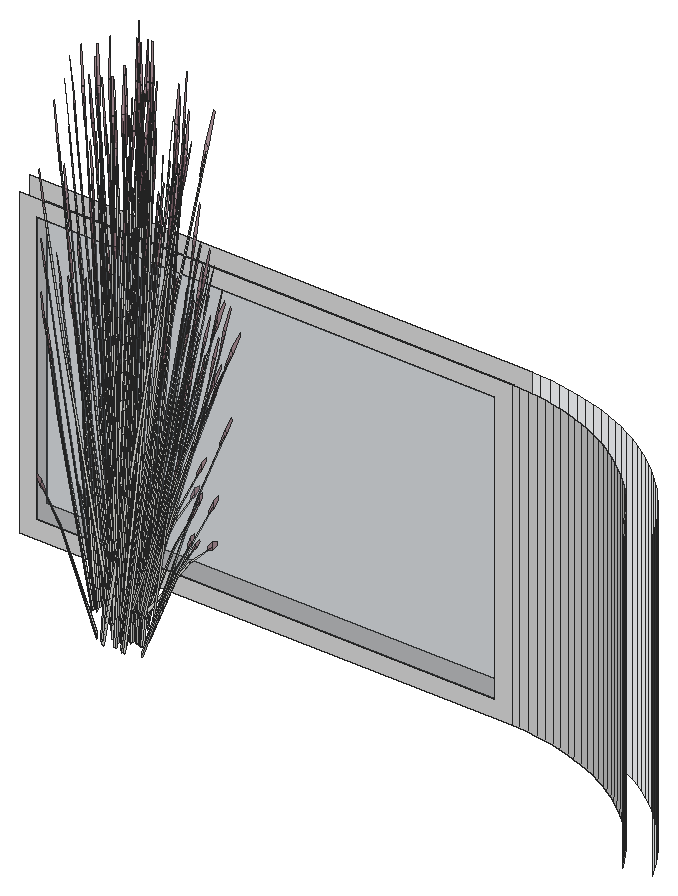
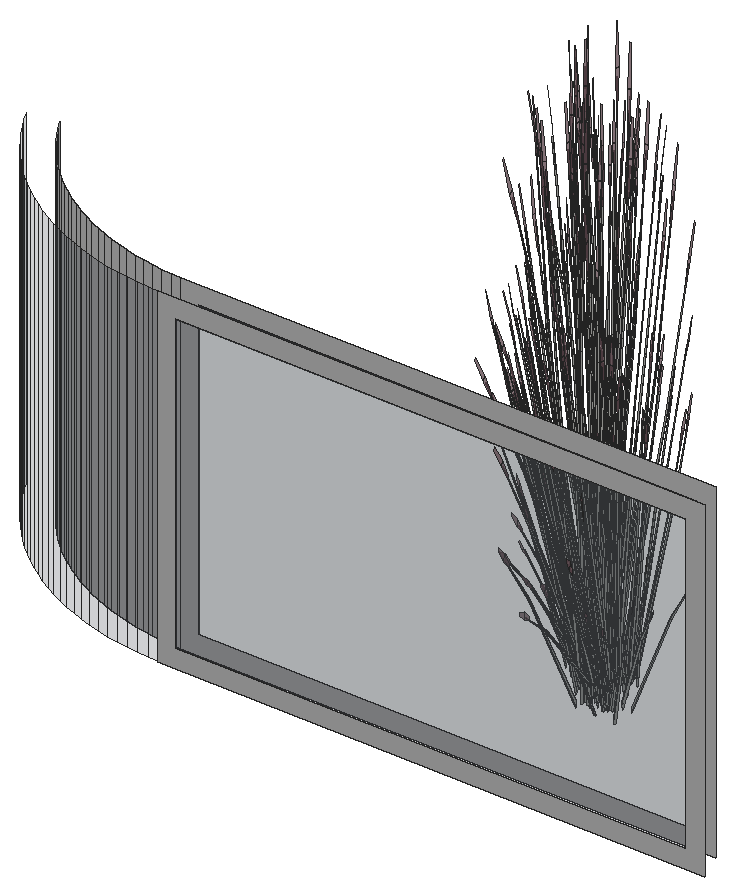
# SketchUp Ruby script. Lengths in inches.
U = 1.inch
M = Sketchup.active_model
def pt(a) = Geom::Point3d.new(a.map { |v| v * U })
def face(e, loops, mat)
  f = e.add_face(loops[0].map { |a| pt(a) })
  loops[1..].each { |l| e.add_face(l.map { |a| pt(a) }).erase! }
  f.material = f.back_material = mat if mat
  f
end
# faces: each face lists its corners as indices into pts; further lists are holes
def faces(e, pts, list, mat = nil) = list.each { |f| face(e, (f[0].is_a?(Array) ? f : [f]).map { |l| l.map { |i| pts[i] } }, mat) }
# xy, xz, yz: faces in a plane at the given z, y or x. An outline is a flat list of corners, or four numbers for a rectangle; further outlines are holes
def ring(l) = l.size == 4 ? [[l[0], l[1]], [l[2], l[1]], [l[2], l[3]], [l[0], l[3]]] : l.each_slice(2).to_a
def flat(e, list, mat, &to3) = list.each { |f| face(e, (f[0].is_a?(Array) ? f : [f]).map { |l| ring(l).map { |u, v| to3.(u, v) } }, mat) }
def xy(e, z, list, mat = nil) = flat(e, list, mat) { |x, y| [x, y, z] }
def xz(e, y, list, mat = nil) = flat(e, list, mat) { |x, z| [x, y, z] }
def yz(e, x, list, mat = nil) = flat(e, list, mat) { |y, z| [x, y, z] }
def lines(e, pts, list) = list.each { |a, b| e.add_line(pt(pts[a]), pt(pts[b])) }
# prism: a flat outline (further loops are holes) pulled along v
def prism(e, loops, v, mat = nil)
  f = face(e, loops, mat); d = Geom::Vector3d.new(v.map { |x| x * U })
  f.pushpull(f.normal.samedirection?(d) ? d.length : -d.length)
end
def box(e, o, s, mat = nil) = prism(e, [[o, [o[0] + s[0], o[1], o[2]], [o[0] + s[0], o[1] + s[1], o[2]], [o[0], o[1] + s[1], o[2]]]], [0, 0, s[2]], mat)
def at(x, y, z, deg = 0) = Geom::Transformation.translation(pt([x, y, z])) * Geom::Transformation.rotation(ORIGIN, Z_AXIS, deg.degrees)
def axes(o, x, y, z) = Geom::Transformation.new([*x, 0, *y, 0, *z, 0, *pt(o).to_a, 1])
def part(name) = M.definitions.add(name)
# library, detail: a bought-in or finely detailed component or shape, given as its bounding box
def library(name, o, s) = part(name).tap { |d| box(d.entities, o, s) }
def detail(e, o, s) = box(e.add_group.entities, o, s)
def put(e, d, t, mat = nil) = e.add_instance(d, t).tap { |i| i.material = mat if mat }
def group(e, t, mat = nil) = e.add_group.tap { |g| g.transformation = t; g.material = mat if mat }.entities
root = M.entities
M.materials.add("Glass_Basic_01").color = [105, 113, 122]
M.materials["Glass_Basic_01"].alpha = 0.25
M.materials.add("LightPink_Translucent").color = [144, 107, 117]
M.materials["LightPink_Translucent"].alpha = 0.75
M.materials.add("M01_Silver_Fog").color = [224, 224, 224]
c1 = part("blade")
p = [[2.15,0.21,22],[0,0.17,0],[0.09,0.45,0],[2.18,0.31,22],[2.29,0.31,22],[0.38,0.45,0],
  [2.48,0.24,33],[2.49,0.24,33],[2.48,0.22,33]]
faces(c1.entities,p,[[0,1,2,3],[4,5,2,3],[6,3,4,7],[8,0,3,6]])
c2 = part("seeds")
p = [[0.3,-0.1,1.38],[-0.01,-0.03,1.59],[-0.01,-0.03,0.03],[0.14,-0.07,-0.07],[0.29,-0.03,3],[0.15,0.01,3.11]]
faces(c2.entities,p,[[0,1,2,3],[1,0,4,5]],"LightPink_Translucent")
c3 = part("blade with seeds")
put(c3.entities,c1,at(0,0,0))
put(c3.entities,c2,axes([2.4,0.25,30.99],[1.5799,-0.05474,1.17369],[-0.12525,1.92788,0.29478],[-0.07173,-0.02425,1.56792]))
xz(root,465.98,[[355.17,648,355.18,684]],"Glass_Basic_01")
xz(root,474,[[275.49,650,329.45,682]],"Glass_Basic_01")
xz(root,474,[[[273.49,648,331.45,684],[275.49,650,329.45,682]]],"M01_Silver_Fog")
xz(root,477,[[274.25,650,329.5,682]],"Glass_Basic_01")
xz(root,477,[[[272.25,648,331.5,684],[274.25,650,329.5,682]]],"M01_Silver_Fog")
yz(root,358.13,[[462.03,648,462.04,684]],"Glass_Basic_01")
p = [[355.6,460.43,648],[356.18,459.47,648],[356.18,459.47,684],[355.6,460.43,684],[359.37,459.91,648],[358.77,460.99,648],
  [358.77,460.99,684],[359.37,459.91,684],[354.98,461.36,648],[354.98,461.36,684],[358.13,462.03,648],[358.13,462.03,684],
  [354.33,462.26,648],[354.33,462.26,684],[358.13,462.04,648],[357.45,463.0625,648],[357.45,463.0625,684],[358.13,462.04,684],
  [353.64,463.14,648],[353.64,463.14,684],[352.92,464,648],[352.92,464,684],[356.73,464.0625,648],[356.73,464.0625,684],
  [352.17,464.83,648],[352.17,464.83,684],[355.97,465.03,648],[355.97,465.03,684],[351.39,465.62,648],[351.39,465.62,684],
  [355.18,465.98,648],[355.18,465.98,684],[350.58,466.39,648],[350.58,466.39,684],[355.17,465.98,648],[354.35,466.89,648],
  [354.35,466.89,684],[355.17,465.98,684],[349.74,467.125,648],[349.74,467.125,684],[353.49,467.76,648],[353.49,467.76,684],
  [348.87,467.83,648],[348.87,467.83,684],[347.97,468.5,648],[347.97,468.5,684],[352.59,468.61,648],[352.59,468.61,684],
  [347.05,469.13,648],[347.05,469.13,684],[351.67,469.42,648],[351.67,469.42,684],[346.11,469.73,648],[346.11,469.73,684],
  [350.71,470.19,648],[350.71,470.19,684],[345.15,470.29,648],[345.15,470.29,684],[349.72,470.93,648],[349.72,470.93,684],
  [344.16,470.82,648],[344.16,470.82,684],[343.16,471.3,648],[343.16,471.3,684],[348.71,471.63,648],[348.71,471.63,684],
  [342.13,471.75,648],[342.13,471.75,684],[347.67,472.29,648],[347.67,472.29,684],[341.09,472.16,648],[341.09,472.16,684],
  [340.04,472.53,648],[340.04,472.53,684],[346.61,472.91,648],[346.61,472.91,684],[338.97,472.86,648],[338.97,472.86,684],
  [337.89,473.15,648],[337.89,473.15,684],[345.52,473.49,648],[345.52,473.49,684],[336.8,473.4,648],[336.8,473.4,684],
  [335.71,473.6,648],[335.71,473.6,684],[344.41,474.03,648],[344.41,474.03,684],[334.6,473.77,648],[334.6,473.77,684],
  [333.49,473.89,648],[333.49,473.89,684],[332.38,473.97,648],[332.38,473.97,684],[331.45,474,648],[331.45,474,684],
  [343.29,474.52,648],[343.29,474.52,684],[342.14,474.97,648],[342.14,474.97,684],[340.98,475.38,648],[340.98,475.38,684],
  [339.8,475.75,648],[339.8,475.75,684],[338.61,476.0625,648],[338.61,476.0625,684],[337.41,476.34,648],[337.41,476.34,684],
  [336.2,476.5625,648],[336.2,476.5625,684],[334.99,476.74,648],[334.99,476.74,684],[333.76,476.88,648],[333.76,476.88,684],
  [332.53,476.97,648],[332.53,476.97,684],[331.5,477,648],[331.5,477,684]]
faces(root,p,[[0,1,2,3],[8,0,3,9],[12,8,9,13],[18,12,13,19],[20,18,19,21],[24,20,21,25],[28,24,25,29],[32,28,29,33],
  [38,32,33,39],[42,38,39,43],[44,42,43,45],[48,44,45,49],[52,48,49,53],[56,52,53,57],[60,56,57,61],[62,60,61,63],
  [66,62,63,67],[70,66,67,71],[72,70,71,73],[76,72,73,77],[78,76,77,79],[82,78,79,83],[84,82,83,85],[88,84,85,89],
  [90,88,89,91],[92,90,91,93],[94,92,93,95]],"M01_Silver_Fog")
faces(root,p,[[4,5,6,7],[5,10,11,6],[14,15,16,17],[15,22,23,16],[22,26,27,23],[26,30,31,27],[34,35,36,37],[35,40,41,36],
  [40,46,47,41],[46,50,51,47],[50,54,55,51],[54,58,59,55],[58,64,65,59],[64,68,69,65],[68,74,75,69],[74,80,81,75],
  [80,86,87,81],[86,96,97,87],[96,98,99,97],[98,100,101,99],[100,102,103,101],[102,104,105,103],[104,106,107,105],[106,108,109,107],
  [108,110,111,109],[110,112,113,111],[112,114,115,113],[114,116,117,115]],"Glass_Basic_01")
put(root,c3,axes([293.05,460.52,652.53],[-0.41757,-0.15024,-0.35414],[0.12179,-0.4383,0.4572],[-0.16812,0.04019,0.87481]))
put(root,c3,axes([291.88,461.33,652.71],[0.06412,0.01444,1.77383],[0.19837,0.47583,-0.16761],[-0.13126,0.12489,0.31391]))
put(root,c3,axes([293.34,460.74,652.68],[-0.13612,0.48987,-0.51099],[-0.46669,-0.16791,-0.3958],[-0.1879,0.04492,0.97773]))
put(root,c3,axes([293.11,460.71,649.49],[0.01274,0.08487,1.76342],[-0.25688,0.44323,-0.26939],[-0.18246,-0.02234,0.30037]))
put(root,c3,axes([292.42,462.84,650.77],[0.2094,-0.24408,1.1486],[0.08263,0.38639,0.84392],[-0.15132,0.06919,0.25299]))
put(root,c3,axes([293.15,460.46,652.73],[0.14195,-0.49104,0.48003],[0.46669,0.16791,0.3958],[-0.18353,0.02951,0.9933]))
put(root,c3,axes([293.32,460.32,653.03],[0.25281,0.48765,-0.1216],[-0.44869,0.23964,-0.67495],[-0.18908,0.06434,1.02557]))
put(root,c3,axes([293.11,460.33,652.73],[-0.18454,-0.3672,0.0643],[0.33652,-0.17973,0.50621],[-0.14834,0.03546,0.77189]))
put(root,c3,axes([293.96,461.35,651.875],[0.1255,-0.16547,1.71376],[0.31687,0.44665,0.13857],[-0.21734,0.2034,0.73262]))
put(root,c3,axes([293.21,461.78,652.53],[-0.43736,0.07697,-0.35414],[-0.11549,-0.43998,0.4572],[-0.12533,0.11818,0.87481]))
put(root,c3,axes([292.97,463.09,649.49],[0.0674,0.0538,1.76342],[0.11428,0.49852,-0.26939],[-0.14937,0.10631,0.30037]))
put(root,c3,axes([293.26,461.6875,652.73],[-0.12461,-0.49565,0.48003],[0.48882,-0.08602,0.3958],[-0.14406,0.11657,0.9933]))
put(root,c3,axes([293.17,461.59,652.73],[-0.34493,-0.22649,0.0643],[0.20082,-0.32253,0.50621],[-0.11059,0.10427,0.77189]))
put(root,c3,axes([293.87,461.76,651.875],[0.09355,-0.18511,1.71376],[0.39247,0.38307,0.13857],[-0.17705,0.23875,0.73262]))
put(root,c3,axes([293.49,460.47,653.05],[0.41757,0.15024,0.35414],[-0.12179,0.4383,-0.4572],[-0.16812,0.04019,0.87481]))
put(root,c3,axes([293.57,461.83,652.68],[0.12908,0.49174,-0.51099],[-0.48882,0.08602,-0.3958],[-0.14008,0.13208,0.97773]))
put(root,c3,axes([292.8,462.72,652.72],[-0.01249,0.10657,1.74944],[0.35444,0.37075,-0.27667],[-0.09279,0.17532,0.14031]))
put(root,c3,axes([294.79,461.48,650.06],[-0.52267,-0.08829,-0.62353],[0.11029,-0.54463,-0.16365],[-0.15598,-0.06599,1.37633]))
put(root,c3,axes([294.1,462.51,650.02],[-0.47024,-0.26927,-0.49651],[0.28107,-0.48284,0],[-0.1071,-0.06133,1.57504]))
put(root,c3,axes([293.34,461.48,653.03],[0.46478,0.29695,-0.1216],[-0.26776,0.43004,-0.67495],[-0.13131,0.14949,1.02557]))
put(root,c3,axes([294.39,462.84,650.375],[-0.31414,0.53965,0],[-0.52557,-0.30095,-0.51607],[-0.1197,-0.06854,1.63711]))
put(root,c3,axes([292.57,462.77,653.65],[0.44338,0.14375,-0.06488],[-0.13639,0.44245,-0.29416],[-0.07252,0.06718,0.97024]))
put(root,c3,axes([293.5625,461.52,653.05],[0.43736,-0.07697,0.35414],[0.11549,0.43998,-0.4572],[-0.12533,0.11818,0.87481]))
put(root,c3,axes([293.8125,463.62,650.59],[0.15856,-0.08496,1.43002],[0.39147,0.25616,-0.30754],[-0.11652,0.22165,0.61141]))
put(root,c3,axes([295.38,461.5625,650.67],[-0.5073,0.35754,-0.29095],[-0.33735,-0.5052,-0.50002],[-0.12516,-0.05131,1.59708]))
put(root,c3,axes([293.98,462.69,652.73],[-0.35779,-0.36745,0.48003],[0.37996,-0.3169,0.3958],[-0.066,0.17239,0.9933]))
put(root,c3,axes([294.23,462.3125,650.03],[-0.11803,-0.46926,-0.30978],[0.46876,-0.13325,0.30978],[-0.0945,-0.05411,1.38974]))
put(root,c3,axes([293.85,462.66,652.73],[-0.4129,-0.02509,0.0643],[0.01132,-0.37891,0.50621],[-0.04321,0.14514,0.77189]))
put(root,c3,axes([293.98,462.8,652.53],[-0.33997,0.28354,-0.35414],[-0.32182,-0.32376,0.4572],[-0.04897,0.1645,0.87481]))
put(root,c3,axes([295.72,461.95,650.06],[-0.33843,0.40479,-0.62353],[-0.42041,-0.36705,-0.16365],[-0.13561,0.10098,1.37633]))
put(root,c3,axes([292.76,463.8125,652.71],[0.057,-0.03251,1.77383],[0.47114,0.21627,-0.16761],[-0.01107,0.18007,0.31391]))
put(root,c3,axes([295.95,461.73,650.46],[-0.49063,-0.43346,-0.25192],[0.41285,-0.48673,0.5513],[-0.13212,0.05071,1.68216]))
put(root,c3,axes([294.2,462.5,653.34],[-0.01307,0.49815,-0.7886],[-0.55054,-0.03346,0.09517],[-0.0581,0.21104,1.11556]))
put(root,c3,axes([294.19,463.9,650.77],[-0.013,-0.32022,1.1486],[0.32493,0.22839,0.84392],[-0.0639,0.15263,0.25299]))
put(root,c3,axes([295.7,461.63,650.21],[-0.54562,0.03324,-0.44739],[-0.04934,-0.55185,0.21531],[-0.09768,0.05593,1.43643]))
put(root,c3,axes([294.66,462.56,650.48],[0.47024,0.26927,0.49651],[-0.28107,0.48284,0],[-0.1071,-0.06133,1.57504]))
put(root,c3,axes([294.02,463.2,651.36],[0.01104,-0.27801,1.54345],[0.49652,0.14685,0.21329],[-0.04302,0.2963,0.72882]))
put(root,c3,axes([295.33,461.72,650.62],[-0.09693,0.48062,0.1448],[-0.47357,-0.08343,-0.41347],[-0.08619,-0.04935,1.26744]))
put(root,c3,axes([296.27,463.06,650.02],[-0.47024,0.26927,-0.49651],[-0.28107,-0.48284,0],[-0.1071,0.06133,1.57504]))
put(root,c3,axes([296.3,462.91,650.19],[-0.31023,-0.54153,-0.05142],[0.52557,-0.30095,0.51607],[-0.12951,0.05156,1.6363]))
put(root,c3,axes([294.3125,462.67,653],[0.35968,0.36185,-0.5672],[-0.37996,0.3169,-0.43934],[-0.05473,0.18385,1.08528]))
put(root,c3,axes([296.16,462.84,650.03],[-0.46876,-0.13325,-0.30978],[0.11803,-0.46926,0.30978],[-0.0945,0.05411,1.38974]))
put(root,c3,axes([294.15,462.4,653.05],[0.33997,-0.28354,0.35414],[0.32182,0.32376,-0.4572],[-0.04897,0.1645,0.87481]))
put(root,c3,axes([296.43,460.84,650.84],[-0.01373,-0.50706,1.41272],[0.62119,0.13144,0.59816],[-0.14692,0.27746,1.3335]))
put(root,c3,axes([293.9375,462.48,653.4],[0.55221,0.02668,-0.13498],[-0.01509,0.50521,-0.74919],[-0.03836,0.19458,1.13838]))
put(root,c3,axes([293.92,463.21,650.82],[0.45645,-0.09537,0.06507],[0.10494,0.38421,-0.86304],[-0.02894,0.19449,0.7736]))
put(root,c3,axes([296.08,461.48,650.67],[0.05855,0.61451,-0.29095],[-0.60981,0.03716,-0.50002],[-0.10738,0.08185,1.59708]))
put(root,c3,axes([294.72,462.15,651.875],[-0.0123,-0.2067,1.71376],[0.53301,0.13712,0.13857],[-0.03297,0.29456,0.73262]))
put(root,c3,axes([295.17,461.26,650.36],[0.63506,0.11347,0.45755],[-0.12924,0.64083,0.17955],[-0.09281,-0.06188,1.58856]))
put(root,c3,axes([295.01,461.14,650.72],[-0.24378,0.48527,0.44739],[-0.50654,-0.23354,-0.21531],[0,-0.11186,1.43643]))
put(root,c3,axes([294.83,462.28,650.47],[0.53992,-0.14294,0.17642],[0.13332,0.53195,0.35086],[-0.04815,-0.07751,1.60407]))
put(root,c3,axes([295.53,462.37,650.2],[-0.50654,-0.24178,0],[0.24378,-0.50239,0],[0,0,1.62707]))
put(root,c3,axes([296.7,462.97,650.375],[0.31414,0.53965,0],[-0.52557,0.30095,-0.51607],[-0.1197,0.06854,1.63711]))
put(root,c3,axes([295.1,463.21,653.0625],[-0.4951,-0.14079,0.53283],[0.1693,-0.46287,0.43934],[0.02975,0.18203,1.10256]))
put(root,c3,axes([294.97,463.24,652.73],[-0.37023,0.18303,0.0643],[-0.18122,-0.33376,0.50621],[0.03575,0.14712,0.77189]))
put(root,c3,axes([296.44,462.3125,650.47],[0.14515,-0.53522,0.17642],[0.53115,0.15146,0.35086],[-0.09175,0.00261,1.60407]))
put(root,c3,axes([296.19,461.6,650.62],[0.37121,0.32357,0.1448],[-0.30963,0.36505,-0.41347],[-0.08619,0.04935,1.26744]))
put(root,c3,axes([296.0625,461.2,650.3],[-0.46736,-0.46353,-0.06131],[0.46764,-0.46381,0],[-0.01632,-0.01619,1.75571]))
put(root,c3,axes([296.19,461.37,650.72],[0.54562,-0.03324,0.44739],[0.04934,0.55185,-0.21531],[-0.09768,0.05593,1.43643]))
put(root,c3,axes([296.32,462.63,650.33],[0.62903,0.17504,0.30756],[-0.15737,0.62568,-0.36492],[-0.10411,0.07831,1.64885]))
put(root,c3,axes([296.59,462.6,650.48],[0.47024,-0.26927,0.49651],[0.28107,0.48284,0],[-0.1071,0.06133,1.57504]))
put(root,c3,axes([295.64,462.16,650.2],[-0.16394,-0.4643,0],[0.46814,-0.1626,0],[0,0,1.54371]))
put(root,c3,axes([295.05,463.14,649.49],[0.08132,-0.0293,1.76342],[0.48914,0.1613,-0.26939],[0.0143,0.18179,0.30037]))
put(root,c3,axes([295.16,463.3,652.53],[-0.15148,0.41415,-0.35414],[-0.44193,-0.12079,0.4572],[0.04052,0.16674,0.87481]))
put(root,c3,axes([296.3,461.24,650.21],[-0.24378,0.48527,-0.44739],[-0.50654,-0.23354,0.21531],[0,0.11186,1.43643]))
put(root,c3,axes([294.84,464.04,652.72],[0.06369,0.08672,1.74944],[0.51399,0.03407,-0.27667],[0.05169,0.19126,0.14031]))
put(root,c3,axes([297.27,460.95,650.47],[-0.39477,-0.39228,0.17642],[0.39783,-0.38049,0.35086],[-0.0436,0.08011,1.60407]))
put(root,c3,axes([295.9,460.72,650.21],[0,-0.62313,0],[0.62828,0,0],[0,0,1.79456]))
put(root,c3,axes([296.22,460.97,650.29],[0,0.62282,-0.05637],[-0.62828,0,0],[0,0.01957,1.79368]))
put(root,c3,axes([295.11,462.87,653.05],[0.15148,-0.41415,0.35414],[0.44193,0.12079,-0.4572],[0.04052,0.16674,0.87481]))
put(root,c3,axes([294.88,459.52,650.47],[-0.14515,0.53522,0.17642],[-0.53115,-0.15146,0.35086],[0.09175,-0.00261,1.60407]))
put(root,c3,axes([295.92,462.18,650.29],[0.21845,0.61869,-0.06012],[-0.62418,0.21679,0],[0.00763,0.02161,1.72173]))
put(root,c3,axes([295.2,462.93,652.98],[0.23981,0.43789,-0.71045],[-0.49365,0.24404,0.08574],[0.05608,0.21158,1.00501]))
put(root,c3,axes([297.72,461.36,650.2],[-0.62797,-0.00431,-0.04976],[0,-0.6019,0.49943],[-0.01973,0.13702,1.58352]))
put(root,c3,axes([296.49,459.55,650.47],[-0.53992,0.14294,0.17642],[-0.13332,-0.53195,0.35086],[0.04815,0.07751,1.60407]))
put(root,c3,axes([295.7,464.34,653.65],[0.34721,-0.30895,-0.06488],[0.31814,0.33837,-0.29416],[0.0224,0.09588,0.97024]))
put(root,c3,axes([295.61,460.33,650.36],[-0.4166,0.48873,0.45755],[-0.49494,-0.43142,0.17955],[0.10044,-0.04877,1.58856]))
put(root,c3,axes([296.32,461.1,650.21],[0.35073,0.34786,0],[-0.35073,0.34786,0],[0,0,1.69266]))
put(root,c3,axes([296.3125,460.69,650.72],[0.24378,-0.48527,0.44739],[0.50654,0.23354,-0.21531],[0,0.11186,1.43643]))
put(root,c3,axes([296.1,462.38,650.2],[0.50654,0.24178,0],[-0.24378,0.50239,0],[0,0,1.74954]))
put(root,c3,axes([295.38,463.02,652.68],[0.49392,0.135,-0.51099],[-0.1693,0.46287,-0.3958],[0.04529,0.18636,0.97773]))
put(root,c3,axes([294.96,463.04,653.03],[0.49168,-0.25073,-0.1216],[0.24162,0.44501,-0.67495],[0.06487,0.18753,1.02557]))
put(root,c3,axes([296.15,460.58,650.38],[-0.63506,-0.11347,0.49198],[0.12924,-0.64083,0.19306],[0.09281,0.06188,1.70813]))
put(root,c3,axes([297.59,461.45,650.03],[-0.35073,0.33601,-0.30978],[-0.35073,-0.33601,0.30978],[0,0.10823,1.38974]))
put(root,c3,axes([296.59,461.39,650.09],[0.18424,0.49308,-0.69212],[-0.53071,0.17758,-0.18165],[0.02036,0.16697,1.52773]))
put(root,c3,axes([296.33,460.86,650.21],[0.56215,0,0],[0,0.55754,0],[0,0,1.78407]))
put(root,c3,axes([295.79,460.25,650.72],[-0.30184,-0.45202,0.44739],[0.45719,-0.31831,-0.21531],[0.09768,0.05593,1.43643]))
put(root,c3,axes([296.53,460.8,650.62],[0.46814,-0.15705,0.1448],[0.16394,0.44848,-0.41347],[0,0.0987,1.26744]))
put(root,c3,axes([296.37,460.84,650.67],[0.56585,0.25696,-0.29095],[-0.27246,0.54236,-0.50002],[0.01778,0.13316,1.59708]))
put(root,c3,axes([297.59,460.96,650.48],[0,-0.53854,0.49651],[0.56215,0,0],[0,0.12266,1.57504]))
put(root,c3,axes([297.83,461.46,650.02],[0,0.53854,-0.49651],[-0.56215,0,0],[0,0.12266,1.57504]))
put(root,c3,axes([296.33,463.09,652.73],[-0.49974,0.12359,0.48003],[-0.08673,-0.48481,0.3958],[0.11753,0.14288,0.9933]))
put(root,c3,axes([296.24,463.19,652.73],[-0.22836,0.34211,0.0643],[-0.3252,-0.19918,0.50621],[0.10513,0.10968,0.77189]))
put(root,c3,axes([295.66,462.0625,651.875],[-0.11485,-0.17291,1.71376],[0.53072,-0.14557,0.13857],[0.11995,0.27145,0.73262]))
put(root,c3,axes([295.99,460.12,650.62],[0.09693,-0.48062,0.1448],[0.47357,0.08343,-0.41347],[0.08619,0.04935,1.26744]))
put(root,c3,axes([296.67,459.28,650.48],[-0.47024,-0.26927,0.49651],[0.28107,-0.48284,0],[0.1071,0.06133,1.57504]))
put(root,c3,axes([296.26,462.09,650.18],[0.5275,-0.18273,-0.19198],[0.18536,0.52636,0.00008],[0.05823,-0.0202,1.73897]))
put(root,c3,axes([296.17,462.8,653.05],[-0.0776,-0.43378,0.35414],[0.44361,-0.11454,-0.4572],[0.11915,0.12431,0.87481]))
put(root,c3,axes([296.27,460.53,650.21],[0.30184,0.45202,-0.44739],[-0.45719,0.31831,0.21531],[0.09768,0.05593,1.43643]))
put(root,c3,axes([296.47,460.3,652.47],[-0.43417,-0.27982,1.38283],[0.45844,-0.43566,0.59665],[0.14008,0.26255,1.33663]))
put(root,c3,axes([295.74,463.4,652.71],[0.00149,-0.0652,1.77383],[0.43058,-0.28766,-0.16761],[0.14956,0.10267,0.31391]))
put(root,c3,axes([297.12,462.58,650.77],[-0.2829,-0.15485,1.1486],[0.36529,-0.15734,0.84392],[0.09853,0.13328,0.25299]))
put(root,c3,axes([296.11,462.41,650.59],[0.00887,-0.17852,1.43002],[0.42372,-0.19941,-0.30754],[0.1308,0.21367,0.61141]))
put(root,c3,axes([297.09,459.53,650.03],[0.11803,0.46926,-0.30978],[-0.46876,0.13325,0.30978],[0.0945,0.05411,1.38974]))
put(root,c3,axes([297.98,461.05,650.375],[0.62828,0,0],[0,0.6019,-0.51607],[0,0.13709,1.63711]))
put(root,c3,axes([295.94,460.27,650.67],[0.5073,-0.35754,-0.29095],[0.33735,0.5052,-0.50002],[0.12516,0.05131,1.59708]))
put(root,c3,axes([297.17,463.28,650.67],[-0.3222,-0.01689,1.0506],[0.21278,-0.35872,0.58006],[0.12729,0.12745,0.8241]))
put(root,c3,axes([296.125,463.02,653.03],[0.2994,-0.46097,-0.1216],[0.43359,0.26557,-0.67495],[0.15072,0.13024,1.02557]))
put(root,c3,axes([294.66,459.96,649.59],[-0.49456,0.21561,1.28929],[-0.15741,-0.61865,0.50096],[0.30369,0.01029,1.46642]))
put(root,c3,axes([296.48,462.79,652.68],[0.4958,-0.12802,-0.51099],[0.08673,0.48481,-0.3958],[0.13317,0.13893,0.97773]))
put(root,c3,axes([297.05,462.21,653.05],[-0.28589,-0.33718,0.35414],[0.32644,-0.31919,-0.4572],[0.16586,0.04856,0.87481]))
put(root,c3,axes([297.22,459.32,650.02],[0.47024,0.26927,-0.49651],[-0.28107,0.48284,0],[0.1071,0.06133,1.57504]))
put(root,c3,axes([297.31,462.52,652.73],[-0.0253,0.40952,0.0643],[-0.38204,-0.01123,0.50621],[0.14634,0.04285,0.77189]))
put(root,c3,axes([297.2,463.16,649.49],[0.03661,-0.07775,1.76342],[0.46087,-0.22898,-0.26939],[0.13972,0.11851,0.30037]))
put(root,c3,axes([297.35,462.39,652.73],[-0.37048,0.35486,0.48003],[-0.31952,-0.37685,0.3958],[0.17382,0.06546,0.9933]))
put(root,c3,axes([298.31,462.4375,651.93],[-0.09617,-0.45271,-0.03492],[0.45453,-0.10408,-0.15832],[0.09492,0.0287,0.52218]))
put(root,c3,axes([297.52,461.27,653.05],[-0.41757,-0.15024,0.35414],[0.12179,-0.4383,-0.4572],[0.16812,-0.04019,0.87481]))
put(root,c3,axes([296.54,460.36,650.06],[0.52267,0.08829,-0.62353],[-0.11029,0.54463,-0.16365],[0.15598,0.06599,1.37633]))
put(root,c3,axes([296.43,461.52,651.875],[-0.18664,-0.09279,1.71376],[0.38624,-0.38925,0.13857],[0.24072,0.1756,0.73262]))
put(root,c3,axes([297.9,461.4,652.73],[0.18454,0.3672,0.0643],[-0.33652,0.17973,0.50621],[0.14834,-0.03546,0.77189]))
put(root,c3,axes([297.46,462.39,652.53],[0.28589,0.33718,-0.35414],[-0.32644,0.31919,0.4572],[0.16586,0.04856,0.87481]))
put(root,c3,axes([297.13,462.43,653.03],[0.0269,-0.54769,-0.1216],[0.50939,0.01497,-0.67495],[0.19618,0.03804,1.02557]))
put(root,c3,axes([297.86,461.27,652.73],[-0.14195,0.49104,0.48003],[-0.46669,-0.16791,0.3958],[0.18353,-0.02951,0.9933]))
put(root,c3,axes([297.57,462.1,652.72],[0.10779,-0.00911,1.74944],[0.29564,-0.41839,-0.27667],[0.19172,0.05523,0.14031]))
put(root,c3,axes([298.85,461.31,650.77],[-0.31044,0.08891,1.1486],[0.14613,-0.36744,0.84392],[0.16469,0.02514,0.25299]))
put(root,c3,axes([297.96,461.22,652.53],[0.41757,0.15024,-0.35414],[-0.12179,0.4383,0.4572],[0.16812,-0.04019,0.87481]))
put(root,c3,axes([297.15,462.16,652.98],[0.50227,0.01297,-0.71045],[-0.03373,0.54602,0.08574],[0.21278,0.05762,1.00501]))
put(root,c3,axes([298.53,460.8,649.49],[-0.02626,-0.08176,1.76342],[0.18213,-0.47826,-0.26939],[0.18372,-0.00688,0.30037]))
put(root,c3,axes([298.7,462.86,652.71],[-0.04543,-0.04715,1.77383],[0.09938,-0.50538,-0.16761],[0.17896,-0.03229,0.31391]))
put(root,c3,axes([296.82,460.67,651.875],[-0.20841,0.0122,1.71376],[0.13825,-0.52864,0.13857],[0.297,0.0327,0.73262]))
put(root,c3,axes([297.59,461.17,652.98],[0.44151,-0.23785,-0.71045],[0.24605,0.4896,0.08574],[0.21333,-0.05562,1.00501]))
put(root,c3,axes([298.27,461.9,650.59],[-0.12101,-0.13245,1.43002],[0.15744,-0.43816,-0.30754],[0.24483,0.05936,0.61141]))
